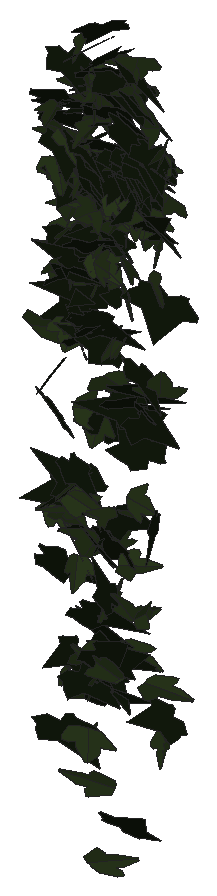
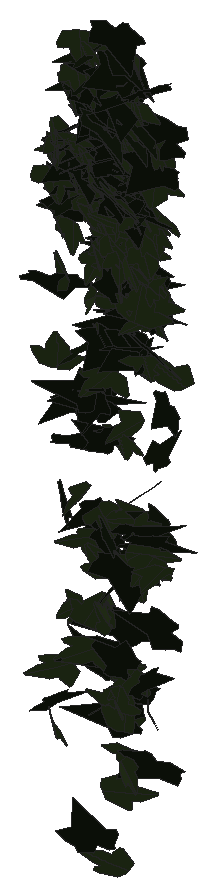
# SketchUp Ruby script. Lengths in millimetres.
U = 1.mm
M = Sketchup.active_model
def pt(a) = Geom::Point3d.new(a.map { |v| v * U })
def face(e, loops, mat)
  f = e.add_face(loops[0].map { |a| pt(a) })
  loops[1..].each { |l| e.add_face(l.map { |a| pt(a) }).erase! }
  f.material = f.back_material = mat if mat
  f
end
# faces: each face lists its corners as indices into pts; further lists are holes
def faces(e, pts, list, mat = nil) = list.each { |f| face(e, (f[0].is_a?(Array) ? f : [f]).map { |l| l.map { |i| pts[i] } }, mat) }
# xy, xz, yz: faces in a plane at the given z, y or x. An outline is a flat list of corners, or four numbers for a rectangle; further outlines are holes
def ring(l) = l.size == 4 ? [[l[0], l[1]], [l[2], l[1]], [l[2], l[3]], [l[0], l[3]]] : l.each_slice(2).to_a
def flat(e, list, mat, &to3) = list.each { |f| face(e, (f[0].is_a?(Array) ? f : [f]).map { |l| ring(l).map { |u, v| to3.(u, v) } }, mat) }
def xy(e, z, list, mat = nil) = flat(e, list, mat) { |x, y| [x, y, z] }
def xz(e, y, list, mat = nil) = flat(e, list, mat) { |x, z| [x, y, z] }
def yz(e, x, list, mat = nil) = flat(e, list, mat) { |y, z| [x, y, z] }
def lines(e, pts, list) = list.each { |a, b| e.add_line(pt(pts[a]), pt(pts[b])) }
# prism: a flat outline (further loops are holes) pulled along v
def prism(e, loops, v, mat = nil)
  f = face(e, loops, mat); d = Geom::Vector3d.new(v.map { |x| x * U })
  f.pushpull(f.normal.samedirection?(d) ? d.length : -d.length)
end
def box(e, o, s, mat = nil) = prism(e, [[o, [o[0] + s[0], o[1], o[2]], [o[0] + s[0], o[1] + s[1], o[2]], [o[0], o[1] + s[1], o[2]]]], [0, 0, s[2]], mat)
def at(x, y, z, deg = 0) = Geom::Transformation.translation(pt([x, y, z])) * Geom::Transformation.rotation(ORIGIN, Z_AXIS, deg.degrees)
def axes(o, x, y, z) = Geom::Transformation.new([*x, 0, *y, 0, *z, 0, *pt(o).to_a, 1])
def part(name) = M.definitions.add(name)
# library, detail: a bought-in or finely detailed component or shape, given as its bounding box
def library(name, o, s) = part(name).tap { |d| box(d.entities, o, s) }
def detail(e, o, s) = box(e.add_group.entities, o, s)
def put(e, d, t, mat = nil) = e.add_instance(d, t).tap { |i| i.material = mat if mat }
def group(e, t, mat = nil) = e.add_group.tap { |g| g.transformation = t; g.material = mat if mat }.entities
root = M.entities
M.materials.add("efeu1").color = [18, 25, 13]
M.materials.add("efeu2").color = [43, 57, 29]
c1 = part("ivyleaf_10")
p = [[0,12.8,-0.8],[-1.5,51.3,-10.9],[-4.9,51,-11.6],[-13.6,26.5,-7.3],[-13.2,15.9,-4.6],[-21.1,19.3,-7.2],
  [-29.5,16.3,-8.3],[-29.2,8.3,-6.2],[-19.7,-9.8,0.5],[-7.6,-13,4],[1,-12.2,5.8],[-0.4,51.1,-11.1],
  [-1.5,51.1,-10.9],[1,-12.4,5.9],[16.9,-12.4,3.5],[35.1,9.1,-5.1],[35,12.9,-6.1],[20.5,16.4,-4.9],
  [15.8,15,-3.8],[15.3,27.6,-7.1],[12.8,31.3,-7.8]]
faces(c1.entities,p,[[0,1,2,3,4,5,6,7,8,9,10],[11,12,0,13,14,15,16,17,18,19,20]],"efeu2")
c2 = part("ivyleaf_9")
p = [[39.1,54.8,31.7],[34.5,51.8,30.2],[-5.3,25.2,17.3],[-17.9,28.3,20.9],[-21.6,21.7,17],[-20.2,4.3,5.3],
  [-22.9,-0.3,2.5],[-17.1,-4,-0.6],[-2,-2.1,-1.2],[-0.7,-15.4,-10.1],[16.6,-22.3,-16.7],[21.1,-15.1,-12.5],
  [32.7,-10.7,-11],[46.1,-1.8,-6.6],[30.8,11.2,3.8]]
faces(c2.entities,p,[[0,1,2,3,4,5,6,7,8,9,10,11,12,13,14]],"efeu1")
put(root,c1,axes([2400.2,995.6,1343.4],[-0.20813,-0.76234,0.19115],[0.03267,-0.19527,-0.76892],[1.49545,-0.10183,0.0434]))
put(root,c1,axes([2386.8,1014.8,668.1],[0.50779,0.7102,0.31257],[0.18965,0.29643,-0.7586],[-1.46454,0.28463,0.01014]))
put(root,c1,axes([2374.9,988.5,973.6],[-0.75812,-0.1554,0.62294],[1.17952,0.09837,0.42084],[-0.31909,0.73284,0.07561]))
put(root,c2,axes([2365,1021.5,579.6],[0.6939,-0.02777,-0.73107],[1.28033,0.33375,0.32282],[0.54722,-0.74565,0.17172]))
put(root,c1,axes([2395.3,1020.8,1130.5],[-0.12051,-0.50996,0.52438],[0.36007,-0.51985,-0.4827],[1.34474,0.0935,0.17624]))
put(root,c1,axes([2407.6,1002.8,1212.5],[-1.25784,0.33329,0.1311],[-0.34632,-0.07549,-0.72543],[-0.58709,-0.66954,0.14705]))
put(root,c2,axes([2409.3,967.5,910.6],[-0.40962,0.40011,-0.72287],[-0.8368,0.57697,0.45026],[1.3313,0.48576,0.0606]))
put(root,c2,axes([2424.6,1024.4,705.3],[-1.13755,-0.28263,0.57223],[-0.94486,-0.28678,-0.6602],[0.76332,-0.77618,0.03556]))
put(root,c1,axes([2410.1,1004.3,1095.5],[-1.59313,0.05836,-0.06664],[-0.1287,-0.01195,0.83895],[0.10889,0.83964,0.01657]))
put(root,c1,axes([2409.1,1001.1,1295.2],[-1.40829,-0.23205,0.0115],[-0.0209,-0.00343,-0.77549],[0.44169,-0.74004,-0.00001]))
put(root,c2,axes([2411.7,994.5,832],[0.42413,-0.69647,0.25184],[-0.06435,0.25316,0.73002],[-1.40805,-0.22136,0.0425]))
put(root,c1,axes([2421.9,1019.9,686.3],[-0.15956,-0.08596,0.86544],[-0.61392,-0.80437,-0.11114],[1.53716,-0.33018,0.04545]))
put(root,c2,axes([2397.9,1001.2,1321.9],[1.16663,0.46137,0.1288],[0.20688,0.06974,-0.76715],[-0.88787,0.62247,-0.00951]))
put(root,c1,axes([2397,1001.8,1053.6],[1.0517,-0.5168,-0.23062],[0.31531,-0.16048,0.75659],[-1.02987,-0.57688,-0.00387]))
put(root,c1,axes([2395.4,1000.1,1240.2],[1.24532,-0.22783,0.34353],[0.60835,-0.12651,-0.69274],[0.49537,0.72812,-0.01287]))
put(root,c1,axes([2415.9,1015.6,1181.6],[-0.75619,-0.6152,0.06936],[-0.04032,-0.06885,-0.73209],[1.17757,-0.39742,0.01947]))
put(root,c1,axes([2406.1,1012.8,674],[-0.85122,-0.49721,-0.40098],[0.49777,0.30404,-0.66873],[1.10908,-0.51806,-0.00762]))
put(root,c2,axes([2437.7,1022.7,715.1],[-1.13693,-0.60988,-0.19757],[-0.20069,-0.17289,0.85254],[-1.20349,0.60498,0.04447]))
put(root,c1,axes([2420,1025.4,1082.8],[-1.67455,0.00114,-0.04807],[-0.09151,-0.024,0.87953],[-0.00033,0.88085,0.02402]))
put(root,c1,axes([2424.1,1002,1137.7],[0.32587,0.61376,-0.36569],[-0.75607,-0.23076,-0.57331],[-1.13014,0.33136,0.2781]))
put(root,c2,axes([2389.5,980.6,1356],[0.92887,-0.02782,0.67419],[1.25399,0.19906,-0.46877],[-0.27691,0.80815,0.13867]))
put(root,c2,axes([2412.1,970.5,708.3],[-0.24309,0.81804,-0.20601],[-0.12105,0.19842,0.82736],[1.60094,0.13922,0.03128]))
put(root,c1,axes([2421.2,1013.9,1225.9],[-1.0349,-0.52106,-0.05839],[0.22094,-0.03761,-0.74546],[0.97313,-0.5456,0.10715]))
put(root,c2,axes([2440.6,999.4,1021.5],[-1.30122,0.35652,0.01757],[-0.03225,0.0055,-0.77107],[-0.67859,-0.6839,0.00296]))
put(root,c1,axes([2419.8,989,1100.2],[-0.53907,-0.75644,-0.39193],[0.34422,0.35022,-0.80664],[1.58446,-0.33344,0.0419]))
put(root,c1,axes([2422.7,991,1307],[-1.37717,0.2994,-0.01837],[0.02537,-0.01582,-0.78304],[-0.57032,-0.72367,0.00952]))
put(root,c2,axes([2413.3,1000.3,1282.2],[-0.28186,-0.73998,0.15713],[0.0082,-0.16094,-0.75384],[1.43971,-0.14395,0.03506]))
put(root,c1,axes([2421.7,1016.6,1202.9],[-1.31298,0.22,-0.17958],[0.23041,-0.19893,-0.70877],[-0.48892,-0.68455,0.14826]))
put(root,c1,axes([2412.4,1009.1,1069.5],[0.26963,0.4354,0.58589],[0.36811,0.5531,-0.45781],[-1.33961,0.23962,-0.00787]))
put(root,c1,axes([2429.3,1011.5,721.7],[0.14006,0.19096,-0.7618],[-0.49991,-0.71509,-0.20462],[-1.40864,0.27277,-0.00313]))
put(root,c2,axes([2434.1,1010.6,1231.1],[-1.27403,-0.3533,-0.10756],[0.20415,0.02707,-0.75648],[0.67257,-0.67746,0.02587]))
put(root,c1,axes([2419.4,1002.2,1090.6],[-0.13592,0.40787,-0.73489],[0.22904,-0.72497,-0.41406],[-1.58313,-0.1399,0.00319]))
put(root,c1,axes([2416.7,999,420.4],[0.54167,-0.31504,0.64025],[0.79603,-0.48482,-0.42448],[1.10029,0.50585,-0.00809]))
put(root,c2,axes([2412.7,993.7,336.9],[-0.50415,-0.3171,-0.72918],[0.89198,0.55862,-0.41319],[1.22252,-0.53835,0.00076]))
put(root,c1,axes([2429,995.7,991.2],[1.13415,0.4652,-0.14589],[-0.2178,-0.0905,-0.75599],[-0.90197,0.6068,-0.0009]))
put(root,c2,axes([2432.6,1000.1,462.8],[0.02628,-0.26501,-0.72541],[0.49575,-0.68142,0.2539],[-1.38373,-0.24917,0.07719]))
put(root,c1,axes([2435,996.3,1229],[0.64965,-0.66357,-0.12192],[-0.117,0.10547,-0.74619],[1.2787,0.34678,-0.00634]))
put(root,c2,axes([2418.8,981.2,1074.9],[0.11026,0.41171,-0.73667],[-0.04492,0.73891,0.4111],[1.60551,-0.0076,0.0621]))
put(root,c1,axes([2412.1,1002.2,1127.1],[1.01266,-0.12201,0.53303],[0.99517,-0.10403,-0.54578],[0.30442,0.74593,0.01107]))
put(root,c1,axes([2436.5,1022.3,1157.1],[-0.00282,-0.7324,0.05146],[0.03705,-0.05148,-0.73215],[1.39686,-0.00011,0.01952]))
put(root,c1,axes([2439.1,1008.9,1228.5],[0.57897,-0.70293,-0.02525],[-0.03194,0.02025,-0.7659],[1.33831,0.30458,-0.00735]))
put(root,c2,axes([2426.1,991.4,1433],[-0.03139,-0.76827,-0.23708],[0.02468,0.23685,-0.76841],[1.53,-0.01958,0.00753]))
put(root,c2,axes([2456.6,985.7,1380.1],[-0.17579,0.78895,0.04557],[-0.21363,0.03231,-0.78703],[-1.48879,-0.09779,0.10755]))
put(root,c2,axes([2448.5,1009.6,1245.4],[0.53202,0.64457,-0.3045],[-0.24911,-0.27511,-0.70251],[-1.33368,0.30851,0.00975]))
put(root,c2,axes([2448.1,1014.6,655],[0.86295,0.6461,-0.32428],[-0.37592,-0.25749,-0.78922],[-1.32349,0.49441,0.01273]))
put(root,c1,axes([2445.9,1018.8,325.6],[0.14251,-0.75365,0.13839],[0.03205,-0.1374,-0.75736],[1.45798,0.07668,0.00312]))
put(root,c1,axes([2434.4,996.7,1298.6],[1.43941,0.15159,0.10744],[0.19821,0.02707,-0.77133],[-0.29284,0.76342,0.00602]))
put(root,c2,axes([2439.7,977.2,1093],[1.27589,0.39495,-0.20021],[-0.32617,-0.10353,-0.77808],[-0.77705,0.69195,-0.00214]))
put(root,c2,axes([2427.1,1004.3,1243.5],[1.08664,-0.50219,-0.11891],[-0.18603,0.06889,-0.76028],[0.96442,0.57912,-0.01267]))
put(root,c2,axes([2475.4,991.5,1060.1],[-0.96441,-0.01581,0.6028],[-1.14728,-0.00682,-0.50692],[0.02929,-0.78746,-0.00771]))
put(root,c2,axes([2463.6,992.1,1364],[-0.05176,0.76113,0.20937],[-0.33199,0.19852,-0.74435],[-1.46524,-0.07187,0.16126]))
put(root,c1,axes([2446.2,1014.3,1144.6],[1.28088,-0.30708,-0.03386],[-0.05707,0.01585,-0.73976],[0.5852,0.67368,0.00197]))
put(root,c2,axes([2433.6,988.3,769.8],[0.53339,-0.66014,-0.30936],[-0.18089,0.29552,-0.7167],[1.37565,0.29482,0.02571]))
put(root,c1,axes([2445.3,989,611.9],[0.36754,0.72146,-0.35683],[-0.1716,-0.34526,-0.74685],[-1.5222,0.21312,-0.00196]))
put(root,c1,axes([2465.2,1007.2,1204.6],[0.96293,0.01664,-0.55127],[-1.04397,0.09291,-0.50064],[0.10906,0.74246,0.075]))
put(root,c2,axes([2455.1,983.5,972.9],[0.22879,-0.56989,0.53563],[0.06901,0.5454,0.57215],[-1.48689,-0.06237,0.10897]))
put(root,c2,axes([2478.6,992.3,1098],[-0.31809,0.06845,0.8358],[-1.59049,0.05731,-0.17181],[-0.13278,-0.85042,0.0557]))
put(root,c2,axes([2430.1,993.5,1143.8],[-0.44051,-0.33322,-0.67897],[0.92497,0.47853,-0.40053],[1.10293,-0.5344,0.06472]))
put(root,c1,axes([2452,986.6,1462.3],[0.54728,-0.76041,-0.04757],[-0.01942,0.04699,-0.81294],[1.44992,0.28765,0.00706]))
put(root,c1,axes([2452.6,1016.5,397.7],[-0.57218,-0.78217,-0.38143],[-0.24248,-0.35964,0.83791],[-1.63835,0.32639,0.0092]))
put(root,c2,axes([2462.6,986.7,611],[0.09718,-0.53417,0.58587],[-0.08044,0.58442,0.53653],[-1.50678,-0.06565,0.00915]))
put(root,c1,axes([2464.9,1007.4,651.5],[-1.38179,-0.4408,0.22937],[-0.37767,-0.11512,-0.84936],[0.86703,-0.75265,-0.00442]))
put(root,c1,axes([2454.1,1020.9,1160.3],[-0.73774,-0.62413,-0.09349],[0.14516,0.06258,-0.73403],[1.19229,-0.3938,0.03152]))
put(root,c2,axes([2437.7,999.3,1299],[0.50517,-0.73695,-0.07388],[-0.02375,0.07402,-0.78318],[1.4094,0.26539,0.01328]))
put(root,c1,axes([2457.3,993.8,1397.3],[-1.43474,-0.22402,-0.07222],[0.12314,0.03576,-0.78628],[0.43071,-0.75646,-0.01578]))
put(root,c1,axes([2470.7,978.5,1404.2],[0.3377,-0.38074,-0.71286],[-0.57906,0.64467,-0.42006],[1.42493,0.35221,-0.00176]))
put(root,c1,axes([2475.9,1000.4,1218.4],[-0.9807,0.27531,0.48439],[-0.9374,0.08332,-0.57132],[-0.49567,-0.70229,0.1221]))
put(root,c1,axes([2459.6,1001.5,1324.5],[-0.02293,-0.56281,0.54498],[0.07582,-0.54478,-0.56172],[1.48909,0.01907,0.03699]))
put(root,c1,axes([2452.5,996,465.8],[-0.61936,-0.51482,-0.62688],[0.58199,0.54776,-0.60859],[1.42995,-0.44592,-0.02383]))
put(root,c2,axes([2476.4,1000.8,1238],[-0.46392,0.71357,-0.08922],[-0.103,-0.11214,-0.74903],[-1.36475,-0.2341,0.08686]))
put(root,c1,axes([2461.8,1003.1,1074],[0.76002,-0.69556,-0.0429],[-0.039,0.0377,-0.80204],[1.32572,0.39986,0.001]))
put(root,c1,axes([2473.4,995.3,1212.5],[-0.19463,0.22738,0.8121],[-0.77422,0.70329,-0.24814],[-1.40596,-0.41876,0.02422]))
put(root,c1,axes([2488.9,992.2,262.5],[-0.34621,0.03462,-0.74937],[-1.39061,-0.18282,0.16892],[-0.32337,0.74914,0.07585]))
put(root,c2,axes([2477.8,985.8,1469.4],[-0.43045,0.73716,-0.26414],[0.03176,-0.27033,-0.76874],[-1.48996,-0.21873,0.05992]))
put(root,c1,axes([2469.4,1020.4,1181.9],[-0.47857,-0.69267,0.08762],[-0.07646,-0.07862,-0.73682],[1.32659,-0.25441,-0.01086]))
put(root,c1,axes([2462.8,1020.1,424.4],[1.46751,0.08981,0.09917],[-0.18776,-0.01018,0.77629],[0.172,-0.77736,0.00129]))
put(root,c2,axes([2469.8,993.8,1401.3],[0.44659,0.75171,0.08399],[-0.01368,0.09015,-0.78676],[-1.43949,0.23235,0.03353]))
put(root,c1,axes([2460.2,981.4,871.3],[0.00021,0.324,0.86638],[-0.06233,0.86584,-0.3238],[-1.75932,-0.03064,0.01158]))
put(root,c2,axes([2455.1,977.4,990.7],[0.7867,0.56215,0.56458],[0.66449,0.44391,-0.69762],[-1.36297,0.54089,-0.01424]))
put(root,c2,axes([2475.4,1012.5,1065.9],[-1.07969,-0.42169,0.28675],[-0.22455,-0.30876,-0.68748],[0.9442,-0.55563,0.1644]))
put(root,c1,axes([2459.3,990.8,334.4],[1.42814,0.13199,0.07397],[0.13706,0.01753,-0.7619],[-0.25325,0.75382,0.00477]))
put(root,c1,axes([2467.3,1008.3,426],[0.3415,-0.67412,0.26593],[0.15402,-0.25361,-0.69749],[1.37058,0.19647,0.01212]))
put(root,c2,axes([2456.2,982.3,437.7],[0.08374,-0.41459,-0.74425],[-0.08891,0.74295,-0.41662],[1.61896,0.06224,0.01562]))
put(root,c1,axes([2479.2,980.4,1202.7],[0.95396,-0.42503,-0.47194],[-0.56529,0.37454,-0.65278],[1.06843,0.57766,0.076]))
put(root,c1,axes([2473.1,1002.5,1127],[0.5458,-0.65018,-0.41383],[-0.09624,0.42473,-0.70234],[1.46366,0.27038,0.10814]))
put(root,c1,axes([2477.5,998.2,1358.6],[1.09416,-0.3788,-0.38537],[-0.45587,0.32573,-0.67752],[0.92187,0.61067,0.12235]))
put(root,c2,axes([2443.2,1024.2,495.5],[0.43575,-0.27836,0.6869],[0.76426,-0.55767,-0.35984],[1.1856,0.4618,-0.0205]))
put(root,c1,axes([2484.8,1013.5,1081.5],[-0.30569,-0.08458,0.73787],[-0.53053,-0.69287,-0.1401],[1.31018,-0.3003,0.11543]))
put(root,c2,axes([2442.6,982,1361.9],[1.05463,-0.133,0.56275],[1.08881,0.23954,-0.50673],[-0.16019,0.75258,0.26074]))
put(root,c2,axes([2459.2,1007.5,1100],[0.92776,0.54379,0.24016],[-0.31924,-0.17213,0.73024],[1.0854,-0.51544,0.0095]))
put(root,c1,axes([2449.8,979.4,719.9],[0.67516,0.17542,0.63125],[1.02161,0.33377,-0.39441],[-0.71495,0.64259,0.03254]))
put(root,c2,axes([2476.9,977.5,1149.8],[0.8359,0.647,-0.13895],[-0.14921,-0.11472,-0.78199],[-1.25058,0.44615,0.00042]))
put(root,c2,axes([2460.8,998.4,1262.1],[0.35122,-0.7603,0.01318],[0.00752,-0.0126,-0.78238],[1.4472,0.18458,0.00087]))
put(root,c1,axes([2472.6,995.9,850.8],[1.34971,-0.32315,0.10312],[0.18131,-0.03962,-0.77932],[0.61959,0.71554,0.00341]))
put(root,c1,axes([2473,995.9,1381.6],[0.55012,-0.69765,0.23424],[0.40332,-0.16209,-0.74428],[1.34129,0.33488,0.12773]))
put(root,c2,axes([2500.1,999.8,978],[-0.61622,-0.63697,-0.36216],[-0.24291,-0.34086,0.71362],[-1.3732,0.34614,0.03628]))
put(root,c1,axes([2451.7,1020.6,1215.7],[0.304,-0.00641,0.72515],[1.37977,-0.01607,-0.15983],[0.03249,0.74236,0.0028]))
put(root,c1,axes([2507.1,983.2,456.9],[-0.75246,0.1074,-0.69101],[-1.28031,0.15841,0.40952],[0.36353,0.7802,0.01197]))
put(root,c2,axes([2460.8,993.3,1239],[0.59768,-0.70545,0.17567],[0.11523,-0.16532,-0.7721],[1.3788,0.31961,-0.01162]))
put(root,c1,axes([2484.1,989,1151],[0.69132,-0.67557,-0.0886],[-0.10941,0.06965,-0.76684],[1.29214,0.36735,-0.01753]))
put(root,c2,axes([2505.2,1006,1258.6],[-0.61934,0.62202,0.30151],[-0.50957,0.19381,-0.68882],[-1.21288,-0.39905,0.13543]))
put(root,c2,axes([2490.6,986.2,1507.2],[0.26933,0.74554,-0.29304],[-0.08818,-0.28946,-0.75881],[-1.52202,0.14869,-0.00789]))
put(root,c2,axes([2450.6,1003.7,398],[0.91732,0.06136,0.68216],[1.29154,0.07009,-0.48579],[-0.17639,0.83231,-0.00938]))
put(root,c1,axes([2457.2,1015.3,1234.7],[0.88965,-0.14604,-0.5731],[1.07367,-0.10918,0.48796],[-0.33788,-0.73146,0.04158]))
put(root,c1,axes([2476.7,993.4,1419.5],[0.1083,0.7923,0.09417],[-0.00075,0.09444,-0.79431],[-1.51852,0.05646,0.00711]))
put(root,c2,axes([2498.9,994,1224.8],[0.11262,0.18429,0.8318],[-0.41295,0.80957,-0.16393],[-1.568,-0.19997,0.10292]))
put(root,c2,axes([2468.2,1026.8,429.7],[0.32798,-0.76287,-0.0972],[-0.03786,0.09515,-0.78209],[1.46315,0.17347,0.00155]))
put(root,c2,axes([2462.4,1004.9,640.8],[0.19937,-0.40209,0.66671],[0.477,-0.6195,-0.41299],[1.40291,0.26777,0.04567]))
put(root,c2,axes([2480.9,1011.6,1248.8],[-0.57747,-0.68109,0.14956],[-0.01209,-0.1604,-0.74334],[1.32708,-0.29783,0.05831]))
put(root,c2,axes([2478.6,984.3,1426.9],[0.96694,0.59704,0.19702],[0.2076,0.16576,-0.7836],[-1.17841,0.5191,0.02362]))
put(root,c1,axes([2491.4,985.7,1388.6],[-1.22316,-0.45043,0.00271],[-0.0042,-0.00157,-0.78481],[0.85726,-0.64269,0.00002]))
put(root,c2,axes([2469.7,986,1306.5],[1.32581,0.30861,0.19682],[0.31622,0.11043,-0.76122],[-0.62072,0.71542,0.0326]))
put(root,c2,axes([2477.7,986.7,1439.8],[0.61114,0.40499,0.72526],[0.72732,0.61837,-0.5145],[-1.40371,0.49673,0.04917]))
put(root,c2,axes([2463,986.6,542],[0.24617,0.15181,-0.77032],[0.79064,0.64923,0.1977],[1.26797,-0.4343,0.02628]))
put(root,c1,axes([2485.5,1014,548],[0.39724,-0.7203,0.22222],[-0.11996,0.21309,0.74993],[-1.4296,-0.21803,-0.00118]))
put(root,c2,axes([2511.6,1005.7,1162.2],[-1.04067,-0.12696,0.51847],[-0.87472,-0.26548,-0.54973],[0.51664,-0.70521,0.11361]))
put(root,c2,axes([2507.4,996.7,1354.8],[-0.029,0.76874,0.18462],[-0.35873,0.17579,-0.74756],[-1.46128,-0.05841,0.17985]))
put(root,c1,axes([2485.4,1019.9,640.1],[-0.29192,-0.74678,0.22942],[0.09835,0.22359,0.76235],[-1.48357,0.16176,0.00539]))
put(root,c2,axes([2474.4,1000.5,1177.3],[0.85802,-0.60687,-0.11641],[-0.10119,0.10547,-0.75574],[1.1717,0.45351,0.01998]))
put(root,c1,axes([2470.4,1020.3,1172.8],[1.0045,-0.1297,0.50611],[0.98073,0.0105,-0.53469],[0.1641,0.73117,0.09746]))
put(root,c1,axes([2493.5,984.8,545.2],[0.56378,-0.6146,0.41791],[-0.35493,0.37403,0.68225],[-1.36925,-0.35001,-0.00477]))
put(root,c2,axes([2495.3,1006.5,694.8],[-0.80424,0.31213,-0.57778],[0.8599,-0.36042,-0.52515],[-0.90701,-0.61846,0.01445]))
put(root,c2,axes([2507.2,983.8,1339.6],[-0.14416,0.78324,0.03306],[-0.00972,0.03272,-0.78689],[-1.49196,-0.07589,0.00193]))
put(root,c2,axes([2467.3,981.9,1023.7],[0.19009,-0.00032,-0.76274],[1.08481,0.51119,0.07443],[0.96461,-0.57483,0.06661]))
put(root,c2,axes([2486.8,994.5,999.2],[0.98588,0.54955,0.22927],[0.27624,0.17819,-0.75505],[-1.0991,0.53773,0.01588]))
put(root,c1,axes([2483,987.7,1119.3],[0.51637,0.61797,0.40989],[0.31995,0.37385,-0.6749],[-1.37457,0.31916,-0.00311]))
put(root,c1,axes([2497.8,972.9,1121.9],[-0.20938,0.53422,0.6029],[-0.35451,0.57514,-0.54361],[-1.49154,-0.21169,0.04457]))
put(root,c1,axes([2501.7,995.6,1180.4],[-0.27532,-0.72566,0.0885],[-0.01153,-0.08902,-0.73985],[1.39126,-0.14434,0.01138]))
put(root,c1,axes([2492.4,1006.7,1229.7],[-1.37033,-0.19323,-0.19757],[0.48389,-0.24714,-0.68489],[0.2061,-0.70454,0.29443]))
put(root,c1,axes([2502.8,1002.3,1274.5],[-1.38493,-0.2288,0.03372],[0.06074,-0.20961,-0.73352],[0.43595,-0.69766,0.20932]))
put(root,c2,axes([2508.3,983.3,573.5],[-0.30789,-0.64486,0.47479],[0.37,0.43827,0.66149],[-1.47848,0.24397,0.06667]))
put(root,c2,axes([2496.5,1006.2,1275.6],[-1.08925,-0.2298,-0.46523],[0.85757,0.12338,-0.61526],[0.48973,-0.72717,0.04263]))
put(root,c2,axes([2487.6,997.7,835.3],[-0.29182,-0.07864,0.76423],[1.34868,0.28655,0.17166],[-0.5648,0.72488,0.01505]))
put(root,c1,axes([2486.1,986,137],[-0.44458,-0.26847,0.6558],[0.8134,0.49742,0.35587],[-1.07577,0.48705,-0.00195]))
put(root,c1,axes([2514.6,991.6,714.7],[-0.86691,-0.60752,0.21564],[-0.23408,-0.17729,-0.75928],[1.20438,-0.47175,0.00765]))
put(root,c1,axes([2509.1,1008.7,1283.8],[-0.11743,-0.7643,-0.04049],[-0.01211,0.04113,-0.76673],[1.45661,-0.06127,-0.00964]))
put(root,c1,axes([2499.9,1018.5,1156.7],[0.88037,-0.55914,0.17539],[0.27531,-0.10758,-0.72448],[1.08076,0.48287,0.04168]))
put(root,c2,axes([2515.5,984.7,1397.6],[0.8526,0.52469,-0.43253],[-0.67358,-0.26235,-0.68482],[-1.10504,0.56475,0.08372]))
put(root,c2,axes([2513.7,1002,1281.4],[-0.75339,0.3905,-0.52634],[0.59864,-0.42625,-0.55281],[-1.09427,-0.50204,0.05995]))
put(root,c1,axes([2501.7,986.7,978.1],[0.41995,-0.82498,0.09562],[-0.00297,0.09853,0.85365],[-1.58062,-0.21937,0.0238]))
put(root,c2,axes([2515.8,978.3,677.1],[0.94492,-0.0131,-0.63003],[-1.19904,0.00724,-0.49663],[0.02625,0.80211,-0.00581]))
put(root,c2,axes([2487.6,983.9,483.7],[0.22001,0.14244,-0.8342],[0.4541,0.8023,0.17006],[1.54528,-0.25605,0.06879]))
put(root,c2,axes([2497.8,978.5,1374.1],[1.32991,0.39802,0.06626],[0.10071,0.04097,-0.80413],[-0.76131,0.70071,0.00938]))
put(root,c2,axes([2488.5,1003.1,464.1],[-0.19046,0.15743,0.80572],[0.98318,-0.61876,0.18506],[1.21432,0.52568,-0.02346]))
put(root,c1,axes([2523.3,1010.7,542.9],[-1.12166,-0.44573,-0.38986],[-0.59742,-0.23124,0.73891],[-0.95564,0.66772,-0.00435]))
put(root,c1,axes([2498.9,1011.6,1259.2],[1.19476,-0.33463,0.27332],[0.57275,-0.00728,-0.70011],[0.59005,0.68465,0.12615]))
put(root,c2,axes([2515,997.3,1278.4],[-1.20843,-0.31036,-0.28574],[0.54818,0.05834,-0.70339],[0.58663,-0.69383,0.06867]))
put(root,c1,axes([2505.8,985.7,934.3],[-0.99479,-0.40509,-0.52109],[0.74537,0.34468,-0.6608],[1.01112,-0.65264,-0.02555]))
put(root,c1,axes([2516.7,1002.6,1126.7],[-1.02269,0.53884,0.05885],[-0.07761,0.04244,-0.76099],[-1.0287,-0.5389,-0.00109]))
put(root,c2,axes([2542,996.3,889.4],[-0.80097,-0.08815,0.66579],[-1.19399,-0.22886,-0.42686],[0.45624,-0.75367,0.05175]))
put(root,c2,axes([2499.3,1020.7,186.3],[1.46761,0.02402,-0.01539],[0.02792,0.02324,0.77117],[0.04658,-0.77093,0.02277]))
put(root,c1,axes([2523.5,986.9,1002.8],[0.61406,-0.70335,-0.12966],[-0.12947,0.11142,-0.77367],[1.35499,0.32939,-0.01517]))
put(root,c2,axes([2514.6,990,1367.7],[1.36513,-0.03176,-0.32894],[-0.61938,0.06873,-0.71629],[0.10931,0.78611,0.04933]))
put(root,c2,axes([2515.3,1007.8,1288.1],[-0.36615,-0.74429,0.01304],[-0.00564,-0.0127,-0.76875],[1.41674,-0.19241,0.00031]))
put(root,c2,axes([2524.5,999.9,902.6],[1.19245,0.0255,-0.47755],[-0.90993,0.01515,-0.62647],[-0.0211,0.78765,0.02751]))
put(root,c1,axes([2535.2,999.8,1198.9],[0.86126,-0.41829,-0.4238],[-0.57716,0.2962,-0.61616],[0.97529,0.54466,0.00961]))
put(root,c1,axes([2516.1,1007.3,1072.6],[-0.35837,0.54769,-0.47254],[0.29446,-0.44649,-0.57916],[-1.34485,-0.24371,-0.00089]))
put(root,c2,axes([2520.1,989,713],[0.26786,0.01105,-0.78214],[-0.43608,0.76043,-0.03049],[1.42342,0.23088,0.13784]))
put(root,c2,axes([2535,1000.5,1281.5],[0.27194,0.74984,-0.03204],[-0.01312,-0.0313,-0.76334],[-1.42835,0.14305,0.00091]))
put(root,c1,axes([2520.9,980.7,1234.1],[0.5152,0.72972,0.18984],[0.13268,0.17662,-0.7783],[-1.42887,0.27951,-0.00382]))
put(root,c1,axes([2531.5,1009.8,1247.9],[0.70443,-0.6507,-0.01195],[-0.00707,0.01163,-0.7486],[1.23861,0.37014,0.00252]))
put(root,c2,axes([2510.8,981.1,891],[0.87261,0.2321,0.66706],[1.05501,0.37457,-0.51134],[-0.83298,0.71756,0.05116]))
put(root,c1,axes([2517.5,1005.2,491.1],[-1.04099,-0.18962,-0.59795],[1.08254,0.18461,-0.57885],[0.50343,-0.78908,0.00826]))
put(root,c2,axes([2525.5,975.4,1360.6],[0.90132,-0.22128,-0.60084],[-0.53941,0.59768,-0.44351],[1.09272,0.47756,0.27666]))
put(root,c1,axes([2532.2,988.8,1212.5],[1.1353,-0.54701,0.10178],[-0.11309,0.08573,0.80903],[-1.05288,-0.59904,0.02285]))
put(root,c1,axes([2535.3,1007.4,1299.4],[0.80459,-0.64464,0.02235],[0.12214,0.01545,-0.76839],[1.22152,0.42307,0.06211]))
put(root,c1,axes([2517.4,1004.3,1280.7],[1.15337,0.03605,0.48638],[0.92422,0.02735,-0.60708],[-0.08608,0.77658,-0.0012]))
put(root,c2,axes([2525.5,988.6,1428.8],[-0.63516,-0.51834,-0.50701],[0.72508,0.34953,-0.60811],[1.17413,-0.49625,0.10126]))
put(root,c1,axes([2547.4,1018.3,1178.7],[-1.1221,0.42707,0.17582],[-0.39745,0.00778,-0.7192],[-0.78399,-0.6152,0.11296]))
put(root,c2,axes([2557.3,1004.8,815.6],[-1.27742,-0.43181,0.12924],[0.21178,0.0659,0.79809],[-0.83129,0.68034,0.00472]))
put(root,c1,axes([2545.9,985.3,1456.6],[0.90493,-0.56022,-0.32375],[-0.27069,0.30144,-0.73051],[1.20133,0.48992,0.07927]))
put(root,c1,axes([2539.5,1000.3,740.8],[-0.17114,0.56013,0.64711],[-0.16254,0.64156,-0.56719],[-1.62075,-0.12349,-0.01145]))
put(root,c2,axes([2527.4,1009.3,1277.8],[0.21664,-0.75777,-0.01867],[0.00506,0.01928,-0.76625],[1.44261,0.11373,0.00549]))
put(root,c2,axes([2513.1,1000.5,905],[0.79771,-0.00437,0.67662],[1.27021,0.13362,-0.41257],[-0.21188,0.78462,0.07403]))
put(root,c1,axes([2540.6,985.2,1411.5],[1.41614,-0.28657,-0.11983],[0.00032,0.31143,-0.74374],[0.59117,0.68631,0.28745]))
put(root,c2,axes([2534.7,1007.2,1280.8],[-0.16064,-0.76088,0.08691],[0.01559,-0.08833,-0.76534],[1.45744,-0.08292,0.01777]))
put(root,c1,axes([2544.8,1004.8,1286.2],[1.29685,-0.32662,-0.07074],[-0.12092,0.0311,-0.75564],[0.62444,0.68436,0.00058]))
put(root,c2,axes([2534.5,1004.2,1298.3],[-0.1108,-0.773,0.08201],[0.01633,-0.08287,-0.77505],[1.47934,-0.05698,0.0147]))
put(root,c1,axes([2547.1,1005,550.2],[0.16974,-0.04022,0.75271],[-0.23077,0.74732,0.0543],[-1.41591,-0.12662,0.08138]))
put(root,c2,axes([2533.6,1003.8,1285],[1.44819,0.06318,0.00846],[0.00572,0.0657,-0.76075],[-0.12117,0.75813,0.06522]))
put(root,c1,axes([2556.7,991.2,1421.1],[-0.85052,-0.6571,0.00396],[-0.01946,0.00216,-0.79461],[1.25047,-0.4469,-0.00967]))
put(root,c1,axes([2556.6,984.8,1471],[-1.1308,-0.54419,-0.00207],[-0.00084,0.00355,-0.8057],[1.03572,-0.59415,-0.00291]))
put(root,c1,axes([2556.6,1002.1,1274.6],[0.19022,-0.7706,-0.10232],[0.08264,0.10853,-0.775],[1.47717,0.09316,0.05653]))
put(root,c2,axes([2535,987.2,1456],[0.83371,-0.68165,-0.06351],[0.03004,0.08544,-0.8081],[1.30258,0.43431,0.05929]))
put(root,c1,axes([2566.6,1008.7,1312.9],[1.23739,-0.00814,-0.4095],[-0.77948,-0.00691,-0.65014],[0.0061,0.76834,-0.01019]))
put(root,c2,axes([2564,1002.7,1236],[-0.02283,-0.02168,-0.77136],[0.23938,-0.76119,0.01944],[-1.449,-0.12541,0.01537]))
put(root,c1,axes([2555.6,1006,1304.8],[1.38278,-0.25353,-0.00901],[-0.01377,0.00663,-0.76951],[0.48262,0.72658,0.00388]))
put(root,c2,axes([2552.3,993.2,1296.1],[1.37852,0.12056,-0.23583],[-0.46442,0.03676,-0.73068],[-0.19599,0.76086,0.07267]))
put(root,c1,axes([2544.4,975.2,651],[-0.07335,-0.13485,-0.74442],[0.98133,0.54077,-0.12466],[1.05363,-0.51305,0.06428]))
put(root,c2,axes([2542.5,986.5,1408.6],[0.98026,-0.61224,-0.09127],[0.01361,0.12461,-0.79554],[1.17802,0.50802,0.08514]))
put(root,c2,axes([2563.7,1003.7,1298.1],[-0.90382,-0.59863,-0.09803],[0.2296,0.02881,-0.76033],[1.13142,-0.48405,0.07598]))
put(root,c1,axes([2561.5,999.5,1218.1],[1.42628,0.05873,0.00738],[0.0128,0.00867,-0.75167],[-0.11193,0.7494,0.00812]))
put(root,c2,axes([2550.8,996.4,960.8],[0.32327,-0.77294,0.08753],[0.06344,-0.08228,-0.79125],[1.47911,0.17246,0.01481]))
put(root,c2,axes([2555.3,996.8,1301.5],[0.08633,-0.74269,-0.27181],[-0.03079,0.27133,-0.74407],[1.50486,0.04816,0.00037]))
put(root,c2,axes([2557.8,991.8,883],[0.14564,-0.30387,-0.73011],[-0.15592,0.72653,-0.31096],[1.49699,0.10524,0.03864]))
put(root,c2,axes([2546.8,992.3,1196.2],[1.57229,0.079,-0.10325],[0.16712,0.15072,0.8179],[0.18246,-0.8188,0.14059]))
put(root,c2,axes([2566.6,1005.5,1308.5],[-0.4214,-0.74001,-0.0517],[0.03919,0.0478,-0.7724],[1.41127,-0.22229,0.00601]))
put(root,c1,axes([2576.7,1009.5,1303.6],[-0.54013,-0.70143,-0.11364],[0.13313,0.0942,-0.7561],[1.3458,-0.29083,0.02919]))
put(root,c2,axes([2583.9,1027.5,391],[0.15338,-0.52699,-0.60206],[0.13764,-0.59783,0.53297],[-1.51655,-0.10755,-0.01252]))
put(root,c2,axes([2557.7,1007.6,1213.3],[0.76264,-0.65686,0.0679],[0.05719,-0.0612,-0.76941],[1.25549,0.40179,-0.00619]))
put(root,c1,axes([2561.2,1017,1094.4],[-0.02473,0.05909,-0.90042],[0.59993,-0.84349,-0.0599],[-1.60918,-0.31538,-0.00849]))
put(root,c1,axes([2591.7,1011,1247.4],[-1.29847,0.14655,0.28738],[-0.5591,-0.00444,-0.69514],[-0.2537,-0.7403,0.06106]))
put(root,c1,axes([2580.7,1008.7,1312.3],[0.32932,-0.63867,-0.38998],[0.07699,0.40767,-0.64969],[1.42212,0.12583,0.12548]))
put(root,c1,axes([2573.4,1005.4,1297.5],[0.68648,0.66502,0.02328],[0.02401,0.01964,-0.75654],[-1.26622,0.36091,-0.00173]))
put(root,c2,axes([2574.9,1004,719.6],[-0.67367,0.24305,-0.78912],[1.24987,-0.43755,-0.42935],[-0.95255,-0.74602,-0.00527]))
put(root,c1,axes([2593.2,976,1382],[0.49233,-0.50635,-0.65736],[-0.52232,0.5976,-0.56832],[1.49034,0.37672,0.01798]))
put(root,c2,axes([2570.6,1001.2,1323.4],[-0.10152,-0.78164,-0.01296],[-0.00592,0.0132,-0.78344],[1.4878,-0.05328,-0.004]))
put(root,c1,axes([2585,1007.1,1327.4],[0.1192,-0.76021,-0.12697],[0.05076,0.12945,-0.7619],[1.46599,0.05733,0.0367]))
put(root,c1,axes([2573.5,1021.5,355.1],[0.86401,-0.50056,0.41985],[0.54168,-0.30867,-0.67576],[1.11923,0.53581,0.00294]))
put(root,c1,axes([2581.2,1007.1,1177.8],[0.50589,-0.60205,0.36787],[0.37566,-0.31396,-0.65645],[1.28918,0.32774,0.04693]))
put(root,c1,axes([2568.7,1008.4,446.5],[-0.61377,-0.23513,-0.68343],[1.12237,0.34705,-0.39768],[0.79523,-0.6713,0.03379]))
put(root,c2,axes([2586.8,1013.7,1082],[-1.16857,-0.64025,-0.18777],[0.24818,0.1351,-0.88708],[1.24535,-0.6277,0.00059]))
put(root,c1,axes([2589.5,997.8,936.2],[-1.06496,-0.54167,-0.08654],[-0.11832,-0.0602,0.77879],[-1.03725,0.56301,0.00001]))
